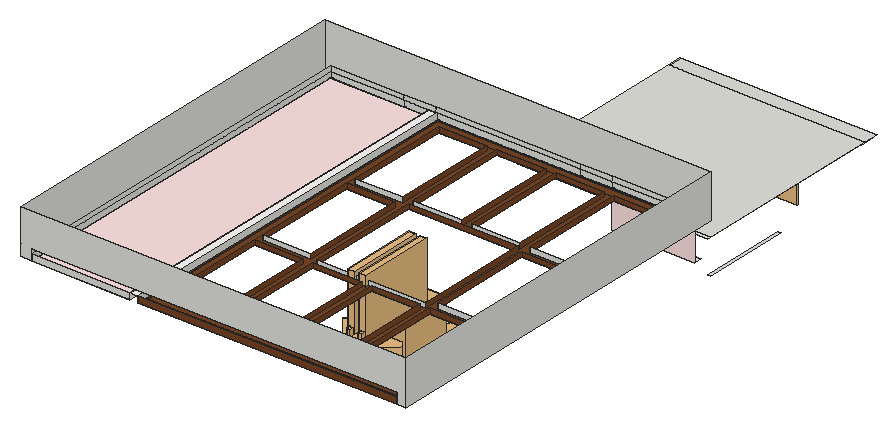
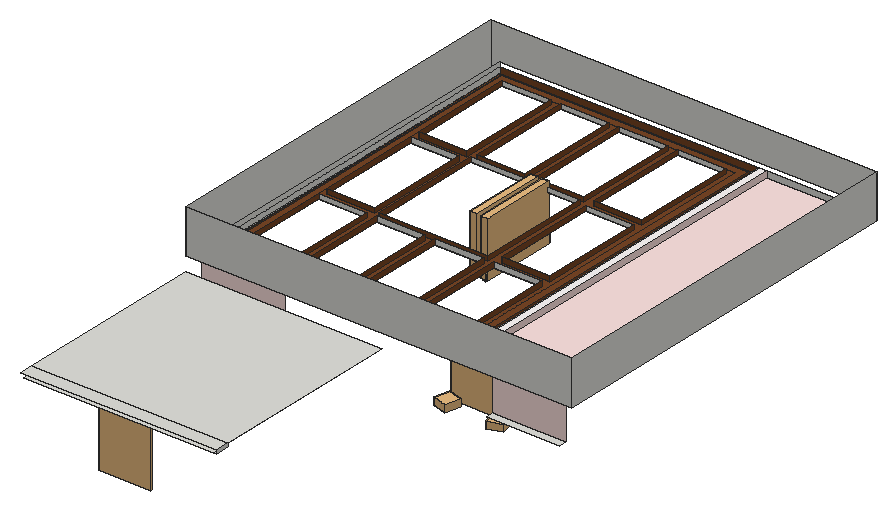
# SketchUp Ruby script. Lengths in inches.
U = 1.inch
M = Sketchup.active_model
def pt(a) = Geom::Point3d.new(a.map { |v| v * U })
def face(e, loops, mat)
  f = e.add_face(loops[0].map { |a| pt(a) })
  loops[1..].each { |l| e.add_face(l.map { |a| pt(a) }).erase! }
  f.material = f.back_material = mat if mat
  f
end
# faces: each face lists its corners as indices into pts; further lists are holes
def faces(e, pts, list, mat = nil) = list.each { |f| face(e, (f[0].is_a?(Array) ? f : [f]).map { |l| l.map { |i| pts[i] } }, mat) }
# xy, xz, yz: faces in a plane at the given z, y or x. An outline is a flat list of corners, or four numbers for a rectangle; further outlines are holes
def ring(l) = l.size == 4 ? [[l[0], l[1]], [l[2], l[1]], [l[2], l[3]], [l[0], l[3]]] : l.each_slice(2).to_a
def flat(e, list, mat, &to3) = list.each { |f| face(e, (f[0].is_a?(Array) ? f : [f]).map { |l| ring(l).map { |u, v| to3.(u, v) } }, mat) }
def xy(e, z, list, mat = nil) = flat(e, list, mat) { |x, y| [x, y, z] }
def xz(e, y, list, mat = nil) = flat(e, list, mat) { |x, z| [x, y, z] }
def yz(e, x, list, mat = nil) = flat(e, list, mat) { |y, z| [x, y, z] }
def lines(e, pts, list) = list.each { |a, b| e.add_line(pt(pts[a]), pt(pts[b])) }
# prism: a flat outline (further loops are holes) pulled along v
def prism(e, loops, v, mat = nil)
  f = face(e, loops, mat); d = Geom::Vector3d.new(v.map { |x| x * U })
  f.pushpull(f.normal.samedirection?(d) ? d.length : -d.length)
end
def box(e, o, s, mat = nil) = prism(e, [[o, [o[0] + s[0], o[1], o[2]], [o[0] + s[0], o[1] + s[1], o[2]], [o[0], o[1] + s[1], o[2]]]], [0, 0, s[2]], mat)
def at(x, y, z, deg = 0) = Geom::Transformation.translation(pt([x, y, z])) * Geom::Transformation.rotation(ORIGIN, Z_AXIS, deg.degrees)
def axes(o, x, y, z) = Geom::Transformation.new([*x, 0, *y, 0, *z, 0, *pt(o).to_a, 1])
def part(name) = M.definitions.add(name)
# library, detail: a bought-in or finely detailed component or shape, given as its bounding box
def library(name, o, s) = part(name).tap { |d| box(d.entities, o, s) }
def detail(e, o, s) = box(e.add_group.entities, o, s)
def put(e, d, t, mat = nil) = e.add_instance(d, t).tap { |i| i.material = mat if mat }
def group(e, t, mat = nil) = e.add_group.tap { |g| g.transformation = t; g.material = mat if mat }.entities
root = M.entities
M.materials.add("[0007_MistyRose]").color = [255, 228, 225]
M.materials.add("[0010_Snow]").color = [255, 250, 250]
M.materials.add("[Wood Veneer 01]").color = [120, 70, 37]
c1 = library("Group13_3",[-10.97,-10.02,0],[21.38,20.04,18.625])
c2 = library("tea cup 06",[-3.13,-3.13,0],[6.26,6.26,3.125])
c3 = library("Utensílios+de+cozinha+(63)",[-13.88,-9.14,0.02],[16.7,15.27,7.73])
c4 = library("Group\#16",[0,0,0],[35.9375,20.89,0.79])
c5 = library("picture+light",[0,0,0],[2.85,31,4.75])
c6 = library("Untitled (24)",[90.5,29.43,0],[57.21,5.13,42.03])
xy(root,109.95,[[286.68,285.5,289,351.1875]])
xy(root,118.49,[[8.87,279.57,63.68,285.5]])
xy(root,118.74,[[219.26,279.57,281.7,285.5]])
xy(root,134.18,[[144.375,285.5,144.375,427.8125,146.93,427.8125,146.93,429.625,147.8,429.625,147.8,427.8125,150.49,427.8125,150.49,429.625,151.36,429.625,151.36,427.8125,154.05,427.8125,154.05,429.625,154.92,429.625,154.92,427.8125,157.62,427.8125,157.62,429.625,158.49,429.625,158.49,427.8125,161.18,427.8125,161.18,429.625,162.05,429.625,162.05,427.8125,164.74,427.8125,164.74,429.625,165.61,429.625,165.61,427.8125,168.3,427.8125,168.3,429.625,169.17,429.625,169.17,427.8125,171.87,427.8125,171.87,429.625,172.74,429.625,172.74,427.8125,175.43,427.8125,175.43,429.625,176.3,429.625,176.3,427.8125,178.99,427.8125,178.99,429.625,179.86,429.625,179.86,427.8125,182.55,427.8125,182.55,429.625,183.42,429.625,183.42,427.8125,186.12,427.8125,186.12,429.625,186.99,429.625,186.99,427.8125,189.68,427.8125,189.68,429.625,190.17,429.625,190.17,427.8125,192.87,427.8125,192.87,429.625,193.36,429.625,193.36,428.0625,196.05,428.0625,196.05,429.625,196.55,429.625,196.55,428.0625,199.24,428.0625,199.24,429.625,199.74,429.625,199.74,428.0625,202.43,428.0625,202.43,429.625,202.92,429.625,202.92,428.0625,205.62,428.0625,205.62,429.625,206.11,429.625,206.11,428.0625,208.8,428.0625,208.8,429.625,209.3,429.625,209.3,428.0625,211.99,428.0625,211.99,429.625,212.49,429.625,212.49,428.0625,215.18,428.0625,215.18,429.625,215.67,429.625,215.67,428.0625,218.37,428.0625,218.37,429.625,218.86,429.625,218.86,428.0625,221.55,428.0625,221.55,429.625,222.05,429.625,222.05,428.0625,224.74,428.0625,224.74,429.625,225.24,429.625,225.24,428.0625,227.93,428.0625,227.93,429.625,228.42,429.625,228.42,428.0625,231.12,428.0625,231.12,429.625,231.61,429.625,231.61,428.0625,234.3,428.0625,234.3,429.625,234.8,429.625,234.8,428.0625,237.49,428.0625,237.49,429.625,237.99,429.625,237.99,428.0625,240.68,428.0625,240.68,429.625,241.17,429.625,241.17,428.0625,243.87,428.0625,243.87,429.625,244.36,429.625,244.36,428.0625,247.05,428.0625,247.05,429.625,247.55,429.625,247.55,428.0625,250.24,428.0625,250.24,429.625,250.86,429.625,250.86,428.375,253.55,428.375,253.55,429.625,254.17,429.625,254.17,428.375,256.87,428.375,256.87,429.625,257.49,429.625,257.49,428.375,260.18,428.375,260.18,429.625,260.8,429.625,260.8,428.375,263.49,428.375,263.49,429.625,264.11,429.625,264.11,428.375,266.8,428.375,266.8,429.625,267.42,429.625,267.42,428.375,270.12,428.375,270.12,429.625,270.74,429.625,270.74,428.375,273.43,428.375,273.43,429.625,274.05,429.625,274.05,428.375,276.74,428.375,276.74,429.625,277.36,429.625,277.36,428.375,280.05,428.375,280.05,429.625,280.67,429.625,280.67,428.375,283.37,428.375,283.37,429.625,283.99,429.625,283.99,428.375,286.68,428.375,286.68,285.5],[144.375,427.8125,146.93,429.625],[147.8,427.8125,150.49,429.625],[151.36,427.8125,154.05,429.625],[154.92,427.8125,157.62,429.625],
  [158.49,427.8125,161.18,429.625],[162.05,427.8125,164.74,429.625],[165.61,427.8125,168.3,429.625],[169.17,427.8125,171.87,429.625],[172.74,427.8125,175.43,429.625],
  [176.3,427.8125,178.99,429.625],[179.86,427.8125,182.55,429.625],[183.42,427.8125,186.12,429.625],[186.99,427.8125,189.68,429.625],[190.17,427.8125,192.87,429.625],
  [193.36,428.0625,196.05,429.625],[196.55,428.0625,199.24,429.625],[199.74,428.0625,202.43,429.625],[202.92,428.0625,205.62,429.625],[206.11,428.0625,208.8,429.625],
  [209.3,428.0625,211.99,429.625],[212.49,428.0625,215.18,429.625],[215.67,428.0625,218.37,429.625],[218.86,428.0625,221.55,429.625],[222.05,428.0625,224.74,429.625],
  [225.24,428.0625,227.93,429.625],[228.42,428.0625,231.12,429.625],[231.61,428.0625,234.3,429.625],[234.8,428.0625,237.49,429.625],[237.99,428.0625,240.68,429.625],
  [241.17,428.0625,243.87,429.625],[244.36,428.0625,247.05,429.625],[247.55,428.0625,250.24,429.625],[250.86,428.375,253.55,429.625],[254.17,428.375,256.87,429.625],
  [257.49,428.375,260.18,429.625],[260.8,428.375,263.49,429.625],[264.11,428.375,266.8,429.625],[267.42,428.375,270.12,429.625],[270.74,428.375,273.43,429.625],
  [274.05,428.375,276.74,429.625],[277.36,428.375,280.05,429.625],[280.67,428.375,283.37,429.625],[283.99,428.375,286.68,429.625],[142.05,429.625,144.375,440.25],
  [144.375,429.625,286.68,440.25]])
xy(root,136.5,[[142.05,285.5,289,429.625],[142.05,429.625,289,440.25]])
xy(root,146.95,[[8.87,0,82.17,279.57]],"[0007_MistyRose]")
xy(root,146.95,[[[88.22,0,281.7,279.57],[92.45,4.23,277.47,275.35]]],"[Wood Veneer 01]")
xy(root,147,[[0,0,0,285.5,289,285.5,289,0,281.7,0,281.7,279.57,8.87,279.57,8.87,0]])
xy(root,149.32,[[[92.45,4.23,277.47,275.35],[97.51,10.67,272.41,268.91]],[[97.51,10.67,272.41,268.91],[144.74,96.75,226.06,182.83],[232.44,14.42,268.65,92.99],[101.27,14.42,137.48,92.99],[101.27,100.5,137.48,179.07],[232.44,100.5,268.65,179.07],[232.44,186.58,268.65,265.15],[101.27,186.58,137.48,265.15],[144.99,14.42,181.2,92.99],[188.72,14.42,224.93,92.99],[188.72,186.58,224.93,265.15],[144.99,186.58,181.2,265.15]]],"[Wood Veneer 01]")
xy(root,151.45,[[82.17,0,88.22,279.57]],"[0010_Snow]")
xz(root,0,[[8.87,146.95,82.17,151.45],[0,147,8.87,147,8.87,155.0625,281.7,155.0625,281.7,147,289,147,289,180.125,0,180.125]])
xz(root,0,[[88.22,146.95,281.7,151.45]],"[Wood Veneer 01]")
xz(root,4.23,[[92.45,146.95,277.47,149.32]])
xz(root,14.42,[[101.27,149.32,137.48,152.95],[144.99,149.32,181.2,152.95],[188.72,149.32,224.93,152.95],[232.44,149.32,268.65,152.95]])
xz(root,92.99,[[101.27,149.32,137.48,152.95],[144.99,149.32,181.2,152.95],[188.72,149.32,224.93,152.95],[232.44,149.32,268.65,152.95]],"[Wood Veneer 01]")
xz(root,96.75,[[144.74,149.32,226.06,152.95]])
xz(root,100.5,[[101.27,149.32,137.48,152.95],[232.44,149.32,268.65,152.95]])
xz(root,179.07,[[101.27,149.32,137.48,152.95],[232.44,149.32,268.65,152.95]],"[Wood Veneer 01]")
xz(root,182.83,[[144.74,149.32,226.06,152.95]],"[Wood Veneer 01]")
xz(root,186.58,[[101.27,149.32,137.48,152.95],[144.99,149.32,181.2,152.95],[188.72,149.32,224.93,152.95],[232.44,149.32,268.65,152.95]])
xz(root,265.15,[[101.27,149.32,137.48,152.95],[144.99,149.32,181.2,152.95],[188.72,149.32,224.93,152.95],[232.44,149.32,268.65,152.95]],"[Wood Veneer 01]")
xz(root,275.35,[[92.45,146.95,277.47,149.32]],"[Wood Veneer 01]")
xz(root,279.57,[[8.87,146.95,63.68,147],[63.68,146.95,82.17,147],[88.22,146.95,195.26,147],[195.26,146.95,219.26,147],[219.26,146.95,281.7,147],
  [8.87,147,63.68,151.45],[63.68,147,82.17,151.45],[87.68,147,88.22,151.45],[88.22,147,195.26,151.45],[195.26,147,219.26,151.45],
  [219.26,147,281.7,151.45],[8.87,151.45,63.68,155.0625],[63.68,151.45,87.68,155.0625],[87.68,151.45,195.26,155.0625],[195.26,151.45,219.26,155.0625],
  [219.26,151.45,281.7,155.0625]])
xz(root,279.57,[[8.87,118.49,63.68,146.95],[219.26,118.74,281.7,146.95],[82.17,147,87.68,151.45]],"[0007_MistyRose]")
xz(root,285.5,[[0,147,289,180.125]])
yz(root,0,[[0,147,285.5,180.125]])
yz(root,8.87,[[0,146.95,279.57,147],[0,147,279.57,151.45],[0,151.45,279.57,155.0625]])
yz(root,82.17,[[0,146.95,279.57,151.45]],"[0007_MistyRose]")
yz(root,88.22,[[0,146.95,279.57,151.45]])
yz(root,92.45,[[4.23,146.95,275.35,149.32]],"[Wood Veneer 01]")
yz(root,101.27,[[14.42,149.32,92.99,152.95],[100.5,149.32,179.07,152.95],[186.58,149.32,265.15,152.95]],"[Wood Veneer 01]")
yz(root,137.48,[[14.42,149.32,92.99,152.95],[100.5,149.32,179.07,152.95],[186.58,149.32,265.15,152.95]],"[Wood Veneer 01]")
yz(root,142.05,[[429.625,134.18,440.25,136.5]])
yz(root,144.74,[[96.75,149.32,182.83,152.95]],"[Wood Veneer 01]")
yz(root,144.99,[[14.42,149.32,92.99,152.95],[186.58,149.32,265.15,152.95]],"[Wood Veneer 01]")
yz(root,181.2,[[14.42,149.32,92.99,152.95],[186.58,149.32,265.15,152.95]],"[Wood Veneer 01]")
yz(root,188.72,[[14.42,149.32,92.99,152.95],[186.58,149.32,265.15,152.95]],"[Wood Veneer 01]")
yz(root,224.93,[[14.42,149.32,92.99,152.95],[186.58,149.32,265.15,152.95]],"[Wood Veneer 01]")
yz(root,226.06,[[96.75,149.32,182.83,152.95]],"[Wood Veneer 01]")
yz(root,232.44,[[14.42,149.32,92.99,152.95],[100.5,149.32,179.07,152.95],[186.58,149.32,265.15,152.95]],"[Wood Veneer 01]")
yz(root,268.65,[[14.42,149.32,92.99,152.95],[100.5,149.32,179.07,152.95],[186.58,149.32,265.15,152.95]],"[Wood Veneer 01]")
yz(root,277.47,[[4.23,146.95,275.35,149.32]],"[Wood Veneer 01]")
yz(root,281.7,[[0,146.95,279.57,147],[0,147,279.57,151.45],[0,151.45,279.57,155.0625]])
yz(root,289,[[0,147,285.5,180.125]])
p = [[2071.65,-901.33,57.89],[2071.65,-899.46,57.89],[2069.91,-901.33,57.89]]
lines(root,p,[[0,1],[1,2],[2,0]])
put(root,c1,axes([142.125,179.57,58.15],[1.7427,0,0],[0,1.87387,0],[0,0,1.68648]))
put(root,c2,axes([117.91,146.14,58.18],[-0.87135,-1.62282,0],[1.50922,-0.93694,0],[0,0,1.68648]))
put(root,c2,axes([117.91,205.82,58.18],[-0.45104,1.81002,0],[-1.68332,-0.48499,0],[0,0,1.68648]))
put(root,c2,axes([156.83,146.14,58.18],[0.87135,-1.62282,0],[-1.50922,-0.93694,0],[0,0,1.68648]))
put(root,c2,axes([156.83,205.82,58.18],[0.45104,1.81002,0],[1.68332,-0.48499,0],[0,0,1.68648]))
put(root,c3,axes([147.45,151,58.17],[1.43201,-1.7651,0],[1.64154,1.5398,0],[0,0,2.10811]))
put(root,c4,axes([204.01,424.41,124.18],[0,0,-1.21],[1.8513,0,0],[0,-1.21,0]))
put(root,c5,axes([170.3,92.55,113.36],[1,0,0],[0,1.9305,0],[0,0,1]))
put(root,c5,axes([178.74,92.55,113.36],[1,0,0],[0,1.9305,0],[0,0,1]))
put(root,c6,at(139.6875,243.07,114.2,-90))
put(root,c6,at(148.125,243.07,114.2,-90))
